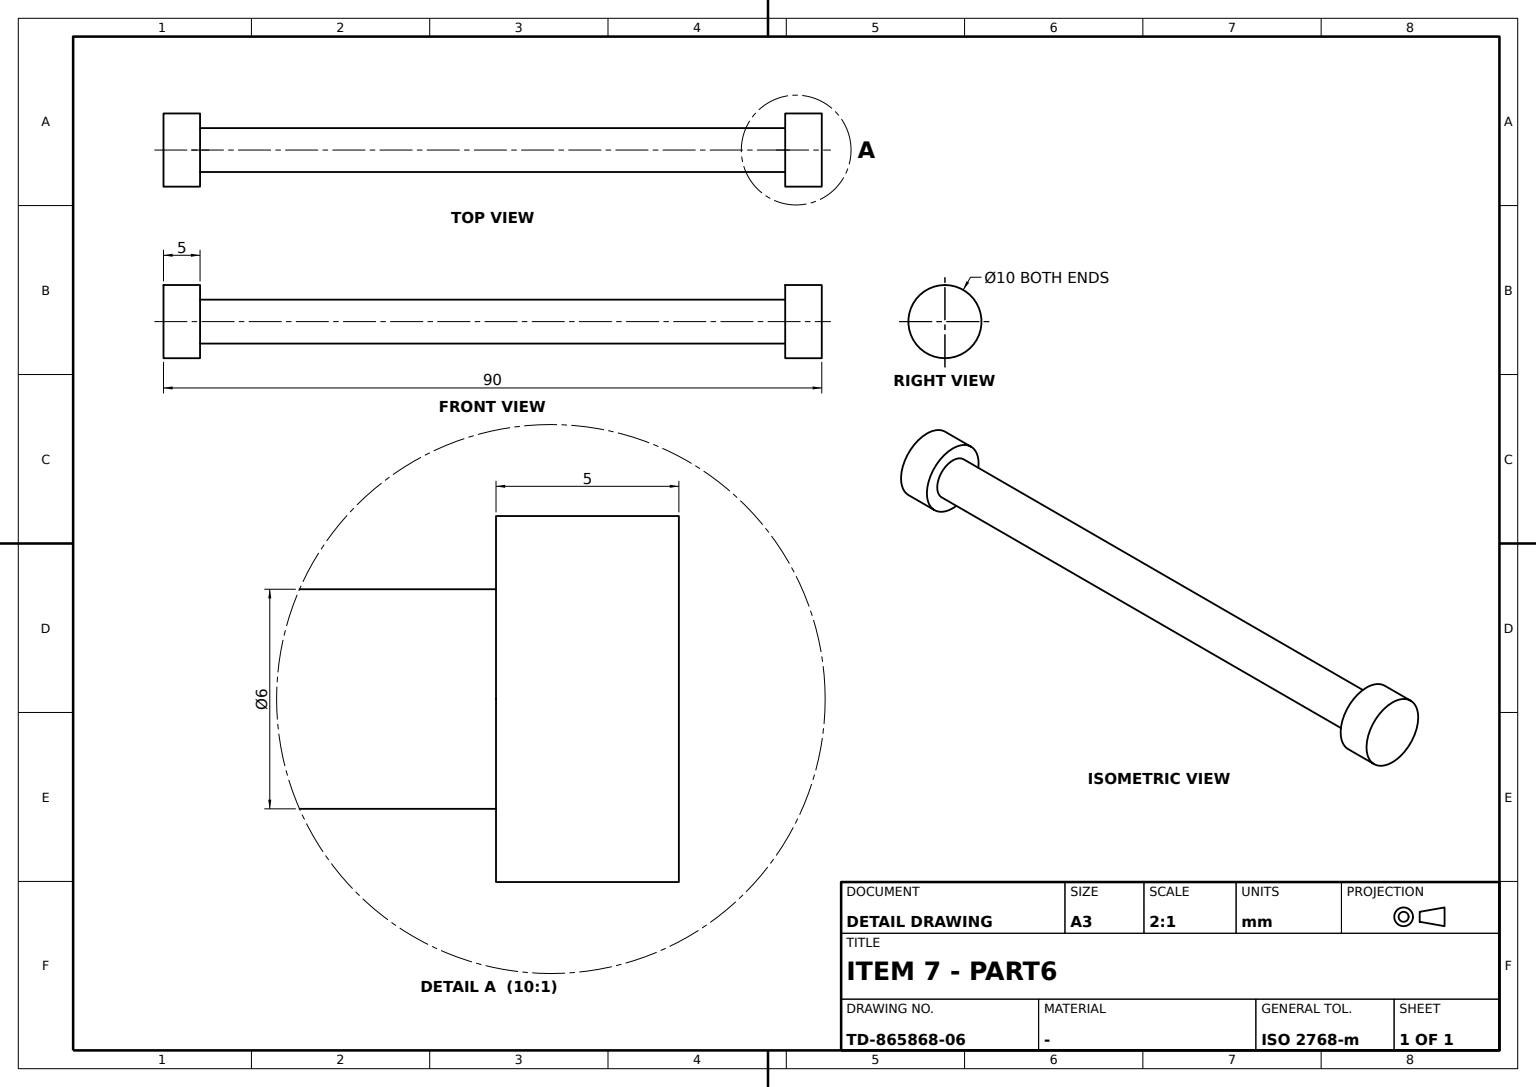
ISO-10303-21;
HEADER;
FILE_DESCRIPTION((''),'2;1');
FILE_NAME('','',(''),(''),'','','');
FILE_SCHEMA(('AUTOMOTIVE_DESIGN'));
ENDSEC;
DATA;
#1=APPLICATION_CONTEXT('');
#2=PRODUCT_CONTEXT('',#1,'mechanical');
#3=PRODUCT('','','',(#2));
#4=PRODUCT_DEFINITION_FORMATION('','',#3);
#5=PRODUCT_DEFINITION_CONTEXT('',#1,'design');
#6=PRODUCT_DEFINITION('','',#4,#5);
#7=PRODUCT_DEFINITION_SHAPE('','',#6);
#8=(LENGTH_UNIT()NAMED_UNIT(*)SI_UNIT(.MILLI.,.METRE.));
#9=(NAMED_UNIT(*)PLANE_ANGLE_UNIT()SI_UNIT($,.RADIAN.));
#10=(NAMED_UNIT(*)SI_UNIT($,.STERADIAN.)SOLID_ANGLE_UNIT());
#11=UNCERTAINTY_MEASURE_WITH_UNIT(LENGTH_MEASURE(0.005),#8,'distance_accuracy_value','');
#12=(GEOMETRIC_REPRESENTATION_CONTEXT(3)GLOBAL_UNCERTAINTY_ASSIGNED_CONTEXT((#11))GLOBAL_UNIT_ASSIGNED_CONTEXT((#8,#9,#10))REPRESENTATION_CONTEXT('',''));
#13=CARTESIAN_POINT('',(0.,85.,3.));
#14=VERTEX_POINT('',#13);
#15=CARTESIAN_POINT('',(0.,85.,0.));
#16=DIRECTION('',(0.,1.,0.));
#17=DIRECTION('',(0.,0.,1.));
#18=AXIS2_PLACEMENT_3D('',#15,#16,#17);
#19=CIRCLE('',#18,3.);
#20=EDGE_CURVE('',#14,#14,#19,.T.);
#21=ORIENTED_EDGE('',*,*,#20,.T.);
#22=EDGE_LOOP('',(#21));
#23=FACE_BOUND('',#22,.T.);
#24=CARTESIAN_POINT('',(0.,85.,5.));
#25=VERTEX_POINT('',#24);
#26=CIRCLE('',#18,5.);
#27=EDGE_CURVE('',#25,#25,#26,.T.);
#28=ORIENTED_EDGE('',*,*,#27,.F.);
#29=EDGE_LOOP('',(#28));
#30=FACE_BOUND('',#29,.T.);
#31=DIRECTION('',(1.,0.,0.));
#32=AXIS2_PLACEMENT_3D('',#13,#16,#31);
#33=PLANE('',#32);
#34=ADVANCED_FACE('',(#23,#30),#33,.F.);
#35=CARTESIAN_POINT('',(0.,5.,3.));
#36=VERTEX_POINT('',#35);
#37=CARTESIAN_POINT('',(0.,5.,0.));
#38=AXIS2_PLACEMENT_3D('',#37,#16,#17);
#39=CIRCLE('',#38,3.);
#40=EDGE_CURVE('',#36,#36,#39,.T.);
#41=ORIENTED_EDGE('',*,*,#40,.T.);
#42=EDGE_LOOP('',(#41));
#43=FACE_BOUND('',#42,.T.);
#44=ORIENTED_EDGE('',*,*,#20,.F.);
#45=EDGE_LOOP('',(#44));
#46=FACE_BOUND('',#45,.T.);
#47=CARTESIAN_POINT('',(0.,45.,0.));
#48=AXIS2_PLACEMENT_3D('',#47,#16,#31);
#49=CYLINDRICAL_SURFACE('',#48,3.);
#50=ADVANCED_FACE('',(#43,#46),#49,.T.);
#51=CARTESIAN_POINT('',(0.,90.,5.));
#52=VERTEX_POINT('',#51);
#53=CARTESIAN_POINT('',(0.,90.,0.));
#54=AXIS2_PLACEMENT_3D('',#53,#16,#17);
#55=CIRCLE('',#54,5.);
#56=EDGE_CURVE('',#52,#52,#55,.T.);
#57=ORIENTED_EDGE('',*,*,#56,.F.);
#58=EDGE_LOOP('',(#57));
#59=FACE_BOUND('',#58,.T.);
#60=ORIENTED_EDGE('',*,*,#27,.T.);
#61=EDGE_LOOP('',(#60));
#62=FACE_BOUND('',#61,.T.);
#63=CYLINDRICAL_SURFACE('',#48,5.);
#64=ADVANCED_FACE('',(#59,#62),#63,.T.);
#65=CARTESIAN_POINT('',(0.,5.,5.));
#66=VERTEX_POINT('',#65);
#67=CIRCLE('',#38,5.);
#68=EDGE_CURVE('',#66,#66,#67,.T.);
#69=ORIENTED_EDGE('',*,*,#68,.T.);
#70=EDGE_LOOP('',(#69));
#71=FACE_BOUND('',#70,.T.);
#72=ORIENTED_EDGE('',*,*,#40,.F.);
#73=EDGE_LOOP('',(#72));
#74=FACE_BOUND('',#73,.T.);
#75=AXIS2_PLACEMENT_3D('',#65,#16,#31);
#76=PLANE('',#75);
#77=ADVANCED_FACE('',(#71,#74),#76,.T.);
#78=CARTESIAN_POINT('',(0.,0.,5.));
#79=VERTEX_POINT('',#78);
#80=CARTESIAN_POINT('',(0.,0.,0.));
#81=AXIS2_PLACEMENT_3D('',#80,#16,#17);
#82=CIRCLE('',#81,5.);
#83=EDGE_CURVE('',#79,#79,#82,.T.);
#84=ORIENTED_EDGE('',*,*,#83,.F.);
#85=EDGE_LOOP('',(#84));
#86=FACE_BOUND('',#85,.T.);
#87=AXIS2_PLACEMENT_3D('',#80,#16,#31);
#88=PLANE('',#87);
#89=ADVANCED_FACE('',(#86),#88,.F.);
#90=ORIENTED_EDGE('',*,*,#56,.T.);
#91=EDGE_LOOP('',(#90));
#92=FACE_BOUND('',#91,.T.);
#93=AXIS2_PLACEMENT_3D('',#51,#16,#31);
#94=PLANE('',#93);
#95=ADVANCED_FACE('',(#92),#94,.T.);
#96=ORIENTED_EDGE('',*,*,#68,.F.);
#97=EDGE_LOOP('',(#96));
#98=FACE_BOUND('',#97,.T.);
#99=ORIENTED_EDGE('',*,*,#83,.T.);
#100=EDGE_LOOP('',(#99));
#101=FACE_BOUND('',#100,.T.);
#102=ADVANCED_FACE('',(#98,#101),#63,.T.);
#103=CLOSED_SHELL('',(#34,#50,#64,#77,#89,#95,#102));
#104=MANIFOLD_SOLID_BREP('',#103);
#105=ADVANCED_BREP_SHAPE_REPRESENTATION('',(#104),#12);
#106=SHAPE_DEFINITION_REPRESENTATION(#7,#105);
ENDSEC;
END-ISO-10303-21;
